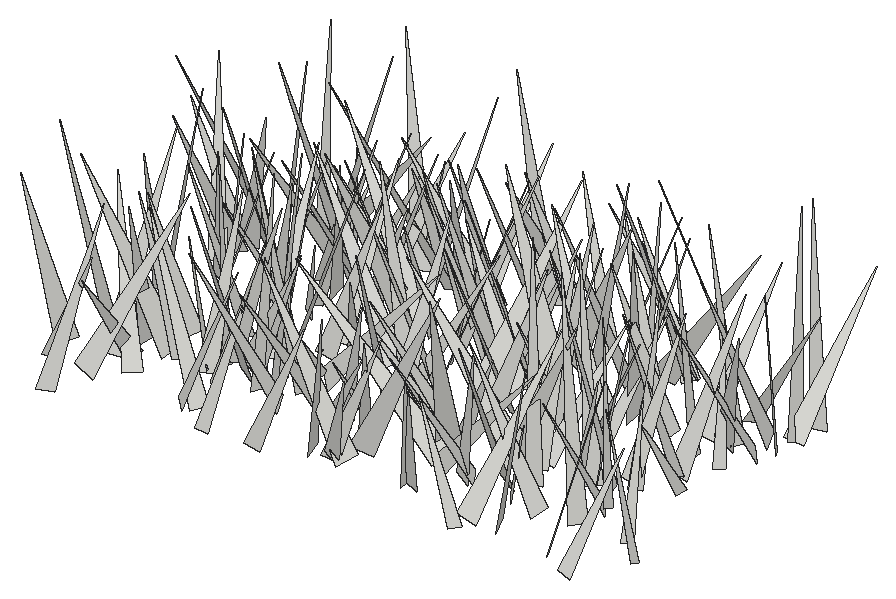
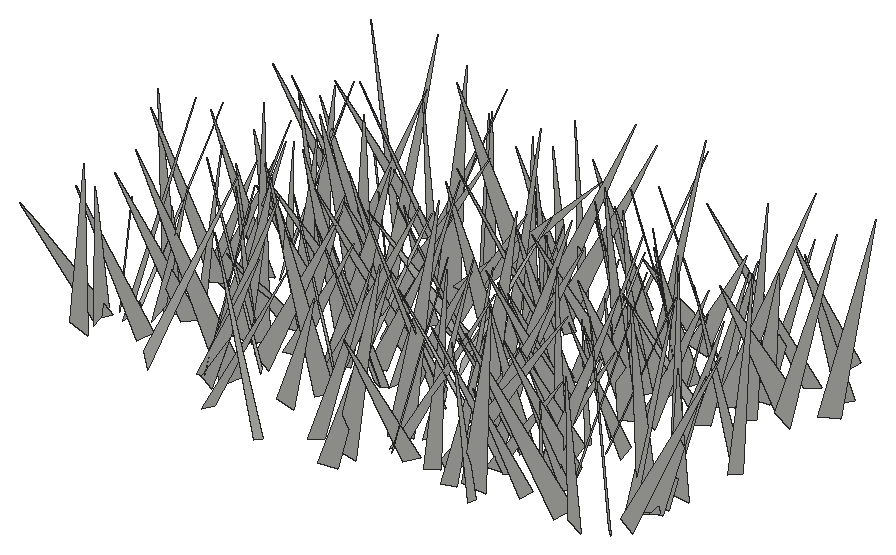
# SketchUp Ruby script. Lengths in inches.
U = 1.inch
M = Sketchup.active_model
def pt(a) = Geom::Point3d.new(a.map { |v| v * U })
def face(e, loops, mat)
  f = e.add_face(loops[0].map { |a| pt(a) })
  loops[1..].each { |l| e.add_face(l.map { |a| pt(a) }).erase! }
  f.material = f.back_material = mat if mat
  f
end
# faces: each face lists its corners as indices into pts; further lists are holes
def faces(e, pts, list, mat = nil) = list.each { |f| face(e, (f[0].is_a?(Array) ? f : [f]).map { |l| l.map { |i| pts[i] } }, mat) }
# xy, xz, yz: faces in a plane at the given z, y or x. An outline is a flat list of corners, or four numbers for a rectangle; further outlines are holes
def ring(l) = l.size == 4 ? [[l[0], l[1]], [l[2], l[1]], [l[2], l[3]], [l[0], l[3]]] : l.each_slice(2).to_a
def flat(e, list, mat, &to3) = list.each { |f| face(e, (f[0].is_a?(Array) ? f : [f]).map { |l| ring(l).map { |u, v| to3.(u, v) } }, mat) }
def xy(e, z, list, mat = nil) = flat(e, list, mat) { |x, y| [x, y, z] }
def xz(e, y, list, mat = nil) = flat(e, list, mat) { |x, z| [x, y, z] }
def yz(e, x, list, mat = nil) = flat(e, list, mat) { |y, z| [x, y, z] }
def lines(e, pts, list) = list.each { |a, b| e.add_line(pt(pts[a]), pt(pts[b])) }
# prism: a flat outline (further loops are holes) pulled along v
def prism(e, loops, v, mat = nil)
  f = face(e, loops, mat); d = Geom::Vector3d.new(v.map { |x| x * U })
  f.pushpull(f.normal.samedirection?(d) ? d.length : -d.length)
end
def box(e, o, s, mat = nil) = prism(e, [[o, [o[0] + s[0], o[1], o[2]], [o[0] + s[0], o[1] + s[1], o[2]], [o[0], o[1] + s[1], o[2]]]], [0, 0, s[2]], mat)
def at(x, y, z, deg = 0) = Geom::Transformation.translation(pt([x, y, z])) * Geom::Transformation.rotation(ORIGIN, Z_AXIS, deg.degrees)
def axes(o, x, y, z) = Geom::Transformation.new([*x, 0, *y, 0, *z, 0, *pt(o).to_a, 1])
def part(name) = M.definitions.add(name)
# library, detail: a bought-in or finely detailed component or shape, given as its bounding box
def library(name, o, s) = part(name).tap { |d| box(d.entities, o, s) }
def detail(e, o, s) = box(e.add_group.entities, o, s)
def put(e, d, t, mat = nil) = e.add_instance(d, t).tap { |i| i.material = mat if mat }
def group(e, t, mat = nil) = e.add_group.tap { |g| g.transformation = t; g.material = mat if mat }.entities
root = M.entities
c1 = part("fur_instance\#9")
p = [[0.8125,0,1.79],[0.67,-0.02,1.48],[0,-0.11,0],[0,0.11,0]]
faces(c1.entities,p,[[0,1,2,3]])
put(root,c1,axes([472.82,384.25,-21.66],[2.29321,-4.71361,1.70331],[-4.8602,-1.63403,2.02152],[1.22385,2.34308,4.83635]))
put(root,c1,axes([457.65,381.76,-21.66],[-5.19171,3.73852,1.55221],[3.028,5.26206,-2.54592],[2.68647,1.29382,5.8693]))
put(root,c1,axes([477.86,386.23,-21.66],[0.93957,-4.99379,0.05949],[-4.70596,-0.86502,1.71172],[1.67197,0.37157,4.78443]))
put(root,c1,axes([489.8,384.13,-21.66],[-1.66543,4.2087,0.7623],[4.0491,1.28782,1.73616],[-1.37806,-1.30242,4.18002]))
put(root,c1,axes([484.14,386.64,-21.66],[-0.53016,-5.209,0.61736],[-4.97847,0.69512,1.58982],[1.65216,0.4231,4.98871]))
put(root,c1,axes([455.08,385.44,-21.66],[2.87453,-4.20489,0.68169],[-4.14129,-2.56592,1.63539],[0.99777,1.46412,4.82385]))
put(root,c1,axes([499.25,383.7,-21.66],[0.30593,5.01742,0.69432],[4.86404,-0.09691,-1.44288],[1.4134,-0.75252,4.8152]))
put(root,c1,axes([476.16,386.43,-21.66],[6.10646,0.88523,1.50787],[1.27518,-6.00248,-1.64024],[-1.19633,-1.87958,5.94829]))
put(root,c1,axes([483.65,386.91,-21.66],[5.31663,-1.02418,0.76649],[-0.77202,-5.18142,-1.56841],[-1.02002,-1.41668,5.18224]))
put(root,c1,axes([491.88,386.17,-21.66],[6.71325,2.37054,1.67819],[2.73448,-6.58312,-1.63968],[-0.97898,-2.13225,6.9281]))
put(root,c1,axes([459.37,388.86,-21.66],[4.70734,-3.12135,0.14145],[-2.64852,-4.12178,-2.81392],[-1.65776,-2.27815,4.89732]))
put(root,c1,axes([478.77,386.71,-21.66],[-7.28796,2.50197,0.93453],[2.66483,6.99355,2.0583],[0.17855,-2.25345,7.42547]))
put(root,c1,axes([465.61,385.81,-21.66],[4.35224,4.23695,0.82253],[4.28263,-4.09432,-1.57033],[0.53605,-1.68972,5.86752]))
put(root,c1,axes([454.67,387.77,-21.66],[4.91943,-4.73173,2.30235],[-4.40019,-5.42749,-1.75256],[-2.8859,0.2095,6.59686]))
put(root,c1,axes([476.04,389.46,-21.66],[2.18391,-6.70079,0.42323],[-6.08063,-2.16263,-2.86325],[-2.84706,-0.52116,6.43986]))
put(root,c1,axes([477.76,386.2,-21.66],[2.95683,-4.48742,1.40063],[-4.613,-2.45121,1.88504],[0.90496,2.16707,5.03253]))
put(root,c1,axes([486.67,390.1,-21.66],[-5.64756,-4.03637,0.24701],[-3.60758,5.22048,2.82493],[1.82721,-2.16853,6.3409]))
put(root,c1,axes([470.7,389.86,-21.66],[-6.78403,-3.28205,0.63683],[-2.89291,6.48484,2.60352],[1.67585,-2.09175,7.07224]))
put(root,c1,axes([488.67,390.94,-21.66],[-2.64275,-7.72517,0.10148],[-7.35563,2.5487,2.46402],[2.36287,-0.70608,7.78402]))
put(root,c1,axes([468.89,383.9,-21.66],[-4.90566,2.32822,0.51514],[1.6552,4.17303,-3.098],[1.71648,2.62995,4.45965]))
put(root,c1,axes([458,385.3,-21.66],[0.84349,7.5995,0.98427],[7.14395,-0.42161,-2.86687],[2.77222,-1.22577,7.08837]))
put(root,c1,axes([477.97,389.6875,-21.66],[0.06322,-6.05576,0.15688],[-5.74231,-0.00994,1.93043],[1.92942,0.16885,5.74018]))
put(root,c1,axes([496.73,385.18,-21.66],[5.00084,3.55671,0.83126],[3.26277,-4.98345,1.69387],[-1.6418,0.92989,5.89825]))
put(root,c1,axes([466.95,386.1,-21.66],[-1.95645,6.57203,0.15793],[5.85701,1.66776,3.15567],[-2.98529,-1.03499,6.08778]))
put(root,c1,axes([478.7,388.26,-21.66],[4.47531,-6.51665,1.20055],[-6.35255,-3.80729,3.0143],[1.88498,2.64087,7.30815]))
put(root,c1,axes([492.91,389.04,-21.66],[-6.35837,1.48,1.02188],[1.69793,6.17763,1.61781],[0.593,-1.81932,6.3247]))
put(root,c1,axes([489.7,385.46,-21.66],[0.36828,7.38641,0.21711],[7.15433,-0.30198,-1.86176],[1.84979,-0.30261,7.15741]))
put(root,c1,axes([486.15,389.51,-21.66],[-1.36067,-5.7583,1.83351],[-5.61411,1.9,1.80082],[2.23642,1.26617,5.63617]))
put(root,c1,axes([466.64,391.48,-21.66],[-3.41876,-7.6362,0.72671],[-7.48826,3.49493,1.49637],[1.66304,0.03883,8.23167]))
put(root,c1,axes([490.25,389.39,-21.66],[3.23905,1.92957,1.10614],[2.22288,-2.8741,-1.49551],[-0.07469,-1.85863,3.46094]))
put(root,c1,axes([474.83,389.55,-21.66],[1.43751,-4.12245,0.23292],[-3.7226,-1.18725,1.96162],[1.78636,0.84328,3.90039]))
put(root,c1,axes([460.84,390.97,-21.66],[-7.92224,1.63819,2.17065],[2.33717,7.51957,2.85498],[1.39032,-3.306,7.56932]))
put(root,c1,axes([458.68,391.3125,-21.66],[6.56004,-2.8558,0.90961],[-2.50702,-6.42798,-2.10074],[-1.6425,-1.59457,6.83935]))
put(root,c1,axes([483.9,390.02,-21.66],[5.26826,5.58359,0.80335],[4.69893,-3.73546,-4.8521],[3.1212,-3.80083,5.9488]))
put(root,c1,axes([465.9,388.77,-21.66],[4.67492,4.49227,1.13099],[4.6277,-4.45606,-1.42912],[0.20972,-1.8104,6.324]))
put(root,c1,axes([483.08,392.04,-21.66],[6.31463,-5.10403,0.36931],[-4.97216,-6.25818,-1.47472],[-1.21044,-0.91981,7.98441]))
put(root,c1,axes([460.55,387.125,-21.66],[-2.20757,6.36235,0.08993],[6.1827,2.12231,1.62203],[-1.50393,-0.61421,6.5362]))
put(root,c1,axes([501.91,387.74,-21.66],[-5.07583,-0.99149,0.0646],[-0.93064,4.62637,-2.11704],[-0.34804,2.08923,4.7186]))
put(root,c1,axes([495.84,392.17,-21.66],[-4.51609,-3.87484,0.43498],[-3.47065,4.29803,2.25393],[1.77713,-1.453,5.5072]))
put(root,c1,axes([477.19,391.42,-21.66],[-3.37323,-1.69913,0.74168],[-1.13548,3.11072,1.96213],[1.46554,-1.50074,3.22735]))
put(root,c1,axes([456.77,389.98,-21.66],[-2.69995,-7.06667,2.40673],[-7.39529,2.18224,-1.88876],[-1.01973,2.88442,7.32531]))
put(root,c1,axes([474.93,391.46,-21.66],[0.27487,-5.90315,0.86813],[-5.62576,0.03312,2.00651],[1.98787,0.91,5.55848]))
put(root,c1,axes([483.4,390.86,-21.66],[-5.86481,5.71927,0.12396],[4.62698,4.63811,4.91939],[-3.36399,-3.59156,6.55024]))
put(root,c1,axes([461.88,390.52,-21.66],[-1.46223,5.38545,2.28823],[5.73287,0.84616,1.67196],[-1.17188,-2.58033,5.32407]))
put(root,c1,axes([493.32,392.2,-21.66],[-0.9776,-5.25666,1.94415],[-5.10339,1.65068,1.89699],[2.31681,1.41798,4.99896]))
put(root,c1,axes([499.82,389.61,-21.66],[-4.30895,1.90574,0.59057],[1.67064,4.21479,-1.41144],[1.09067,1.07302,4.49519]))
put(root,c1,axes([467.54,391.4,-21.66],[3.43659,4.37627,1.35344],[4.55407,-3.08156,-1.59944],[0.49399,-2.03617,5.32951]))
put(root,c1,axes([464.3125,390.48,-21.66],[-4.28089,-1.18354,0.47624],[-1.27514,3.91753,-1.72642],[-0.03977,1.79046,4.09221]))
put(root,c1,axes([476.07,394.37,-21.66],[-2.59583,-7.17613,0.91864],[-6.91744,2.74775,1.9178],[2.11891,0.17907,7.38629]))
put(root,c1,axes([495.76,389.51,-21.66],[-8.22184,1.12863,0.67504],[0.91948,7.98903,-2.15825],[0.94024,2.05661,8.01339]))
put(root,c1,axes([465.83,392.55,-21.66],[0.54416,-5.67013,1.84078],[-5.27926,0.40028,2.79359],[2.76917,1.87733,4.9641]))
put(root,c1,axes([470.54,394.35,-21.66],[3.27584,-2.78093,0.2499],[-2.38988,-2.99185,-1.96583],[-1.44378,-1.35736,3.82103]))
put(root,c1,axes([464.33,390.125,-21.66],[-4.85985,3.92503,1.53679],[3.59209,5.08366,-1.6245],[2.20555,0.36911,6.032]))
put(root,c1,axes([468.42,390.41,-21.66],[-7.01527,0.64484,2.20419],[0.06996,7.14138,-1.86657],[2.29551,1.75305,6.79307]))
put(root,c1,axes([457.87,388.16,-21.66],[-6.65412,4.03174,0.74119],[3.28122,6.08544,-3.64454],[2.45722,2.79179,6.87384]))
put(root,c1,axes([464.7,392.25,-21.66],[5.22316,-4.20753,1.34718],[-4.41725,-5.01042,1.47756],[-0.07792,1.998,6.54228]))
put(root,c1,axes([460.52,393.67,-21.66],[-5.0365,1.95588,2.0654],[2.56555,4.93734,1.5806],[1.22852,-2.29236,5.16658]))
put(root,c1,axes([481.3125,394.34,-21.66],[0.83306,-5.07313,1.39633],[-4.3947,-1.44829,-2.63999],[-2.89363,0.73905,4.41148]))
put(root,c1,axes([469.78,390.22,-21.66],[4.59054,6.55576,1.84003],[6.00661,-4.94402,2.62946],[-3.20693,0.124,7.5589]))
put(root,c1,axes([486.77,394,-21.66],[2.93254,-6.52755,1.0505],[-6.19008,-2.30697,2.94501],[2.32281,2.09313,6.52193]))
put(root,c1,axes([464.77,391.67,-21.66],[-6.75602,-0.97126,1.58692],[-1.43223,6.52998,-2.10085],[1.1876,2.34979,6.49412]))
put(root,c1,axes([464.48,391.13,-21.66],[5.18637,5.57386,2.23152],[5.04396,-5.64447,2.37581],[-3.2567,0.13438,7.23339]))
put(root,c1,axes([470.87,391.87,-21.66],[-7.866,-1.33504,0.19154],[-1.32695,7.45779,-2.51268],[-0.24134,2.50839,7.5725]))
put(root,c1,axes([486.14,394.83,-21.66],[-7.10232,2.48969,0.17848],[2.39972,6.66255,2.55443],[-0.68683,-2.46683,7.07929]))
put(root,c1,axes([482.45,394.32,-21.66],[1.69765,-3.69471,0.41656],[-3.54176,-1.46758,1.41724],[1.13153,0.9496,3.81108]))
put(root,c1,axes([470.97,394.23,-21.66],[5.03462,6.0848,0.40692],[5.07887,-3.8915,-4.64748],[3.37572,-3.22012,6.38538]))
put(root,c1,axes([478.5625,395.4,-21.66],[-4.09373,-0.36711,0.23804],[-0.24891,3.79616,1.57392],[0.35983,-1.55061,3.79686]))
put(root,c1,axes([490.3,391.76,-21.66],[1.13757,8.04859,1.54719],[7.76789,-1.55698,2.3882],[-2.61411,-1.12413,7.76984]))
put(root,c1,axes([487.18,392.28,-21.66],[-2.89965,3.32427,1.06428],[2.78447,3.03733,-1.90073],[2.1048,0.5615,3.98069]))
put(root,c1,axes([496,392.39,-21.66],[-6.18556,-0.57175,1.0735],[-0.94708,5.75521,-2.39186],[0.76312,2.5082,5.73298]))
put(root,c1,axes([468.7,392.64,-21.66],[-4.6642,0.46344,0.8289],[0.1067,4.38406,-1.85075],[0.94364,1.79496,4.30631]))
put(root,c1,axes([464.67,396.26,-21.66],[0.15208,-7.64456,1.76209],[-7.47072,0.39677,2.36609],[2.3943,1.72356,7.27077]))
put(root,c1,axes([494.63,394.7,-21.66],[-7.44301,-3.63877,0.95843],[-3.76282,7.20814,-1.85509],[0.01898,2.08796,8.0745]))
put(root,c1,axes([469.61,393.62,-21.66],[-7.1733,-2.93015,0.73361],[-2.97558,6.52972,-3.01478],[-0.51951,3.05896,7.13815]))
put(root,c1,axes([498.42,396.97,-21.66],[2.63611,-2.6678,0.56163],[-2.26437,-2.5776,-1.61563],[-1.51829,-0.78771,3.38467]))
put(root,c1,axes([489.14,393.42,-21.66],[-5.55671,4.70477,2.20019],[4.40361,5.97611,-1.65743],[2.7539,-0.06297,7.08977]))
put(root,c1,axes([470.57,397.75,-21.66],[5.43533,-0.93824,0.08866],[-0.80913,-4.91198,-2.3767],[-0.48317,-2.32876,4.97739]))
put(root,c1,axes([454.73,397.4375,-21.66],[6.40589,-1.32849,1.4611],[-0.83624,-6.31798,-2.07823],[-1.78897,-1.80373,6.20333]))
put(root,c1,axes([463.44,395.63,-21.66],[-0.2537,5.53184,2.90433],[5.7111,-0.97344,2.35297],[-2.53371,-2.74807,5.0129]))
put(root,c1,axes([469.34,391.5625,-21.66],[6.78257,3.66457,1.14232],[2.83952,-6.35069,3.51329],[-2.58286,2.6414,6.86216]))
put(root,c1,axes([462.27,392.2,-21.66],[5.32818,4.49942,0.50618],[3.89144,-4.95023,3.04014],[-2.31467,2.03493,6.2763]))
put(root,c1,axes([493.37,394.1,-21.66],[-7.58228,1.17889,0.51367],[1.00041,7.33787,-2.07353],[0.80796,1.97752,7.38791]))
put(root,c1,axes([476.41,394.98,-21.66],[-2.09917,6.50868,2.06271],[6.47308,2.58358,-1.56477],[2.17184,-1.40938,6.65739]))
put(root,c1,axes([493.51,394.16,-21.66],[3.73526,4.02595,0.93613],[3.5763,-3.78049,1.98866],[-2.07237,0.73241,5.11915]))
put(root,c1,axes([489.04,394.6,-21.66],[-0.72981,5.66267,0.18679],[5.27184,0.7477,-2.06932],[2.0757,0.09199,5.32132]))
put(root,c1,axes([468.97,396.73,-21.66],[2.35297,-5.60644,2.50548],[-6.03434,-1.6135,2.05656],[1.13856,3.03489,5.72182]))
put(root,c1,axes([494.92,396.01,-21.66],[0.03903,6.40601,1.64221],[6.43648,0.34027,-1.48032],[1.51842,-1.60705,6.23275]))
put(root,c1,axes([491.09,395.7,-21.66],[4.64309,0.99306,0.50279],[0.80416,-4.48393,1.43003],[-0.7696,1.30595,4.52764]))
put(root,c1,axes([456.37,395.5,-21.66],[6.51752,3.06728,2.32468],[2.5593,-6.86862,1.88745],[-2.87443,0.8392,6.95153]))
put(root,c1,axes([466.09,394.17,-21.66],[-5.16112,5.15909,0.10388],[4.87926,4.92701,-2.27629],[1.67923,1.54029,6.93338]))
put(root,c1,axes([463.09,400.33,-21.66],[-4.74866,-3.13825,0.27488],[-2.86364,4.50737,1.98925],[1.31291,-1.51952,5.33303]))
put(root,c1,axes([483.28,398.32,-21.66],[-3.66042,-4.84933,0.70173],[-4.78346,3.34689,-1.82316],[-1.06154,1.63996,5.79575]))
put(root,c1,axes([482.21,397.54,-21.66],[1.25839,-5.65908,2.69216],[-6.0262,-0.33916,2.10388],[1.71982,2.95233,5.40207]))
put(root,c1,axes([477.375,397.82,-21.66],[-7.14593,-4.06809,0.00282],[-3.91681,6.87864,-2.22635],[-1.09909,1.93614,7.91562]))
put(root,c1,axes([476.01,397.3,-21.66],[3.46284,5.45761,0.55951],[5.19477,-3.049,-2.40992],[1.76435,-1.73432,5.99742]))
put(root,c1,axes([457.36,400.3,-21.66],[-1.15928,-6.64992,1.1524],[-6.36185,1.46707,2.06591],[2.25307,0.72087,6.42631]))
put(root,c1,axes([486.22,399.79,-21.66],[-4.22859,-0.79072,0.99748],[-0.41595,4.12901,1.5098],[1.20299,-1.35177,4.02824]))
put(root,c1,axes([495.81,395.41,-21.66],[-6.32088,1.55628,0.92222],[1.03646,5.86264,-2.78949],[1.48264,2.53644,5.88169]))
put(root,c1,axes([496.86,398.52,-21.66],[-1.92463,-5.23066,1.71698],[-5.26178,1.21283,-2.20335],[-1.6191,2.27625,5.1195]))
put(root,c1,axes([474.71,398.29,-21.66],[-1.73257,6.85044,2.42635],[7.20837,1.30251,1.46979],[-0.92468,-2.68187,6.91158]))
put(root,c1,axes([464.72,400.32,-21.66],[-1.05562,-3.90874,0.84941],[-3.49411,1.32871,1.77194],[1.94702,0.26528,3.64044]))
put(root,c1,axes([473.16,398.65,-21.66],[-5.71693,5.39586,0.3581],[5.20349,5.34707,2.50186],[-1.47216,-2.05434,7.45247]))
put(root,c1,axes([478.94,394.9,-21.66],[6.66219,5.05954,0.23915],[4.47229,-6.06129,3.64695],[-2.37798,2.77537,7.52884]))
put(root,c1,axes([486.45,398.26,-21.66],[6.53232,-2.04401,3.08815],[-2.89411,-6.72439,1.67109],[-2.31057,2.64395,6.63752]))
put(root,c1,axes([464.46,398.28,-21.66],[3.7445,3.22853,1.26331],[2.91821,-3.9391,1.41711],[-1.87174,0.31742,4.73672]))
put(root,c1,axes([468.5625,397.27,-21.66],[5.48783,2.36239,1.1528],[1.72376,-5.24883,2.55038],[-1.98455,1.97355,5.40302]))
put(root,c1,axes([496.82,398.58,-21.66],[0.16958,6.97336,1.46095],[6.91324,0.19239,-1.72074],[1.72314,-1.45812,6.75984]))
put(root,c1,axes([479.39,401.86,-21.66],[-7.48109,-1.28394,1.71532],[-0.94889,7.57103,1.5286],[1.92105,-1.26035,7.43496]))
put(root,c1,axes([499.0625,403.91,-21.66],[-5.37416,-4.85351,0.14678],[-4.51514,5.07548,2.5125],[1.7865,-1.77274,6.79157]))
put(root,c1,axes([482.9375,401.17,-21.66],[-5.86461,-3.9483,0.52207],[-3.9663,5.70596,-1.40208],[-0.36068,1.452,6.92942]))
put(root,c1,axes([496.57,403.71,-21.66],[-0.05965,-7.49908,0.31223],[-6.76708,0.1888,3.24163],[3.24657,0.25574,6.76251]))
put(root,c1,axes([493.22,402.39,-21.66],[-6.6748,0.96554,1.83268],[1.43583,6.61336,1.7452],[1.49311,-2.0433,6.51456]))
put(root,c1,axes([489.83,402.99,-21.66],[7.80174,-0.94154,1.76979],[-0.49694,-7.7978,-1.95786],[-1.94209,-1.78708,7.61055]))
put(root,c1,axes([469.38,404.48,-21.66],[6.1806,-4.85252,1.92283],[-3.89661,-6.27237,-3.30423],[-3.47285,-1.59827,7.12944]))
put(root,c1,axes([468.61,398.66,-21.66],[-3.2571,5.60614,0.8435],[5.30317,3.35677,-1.83235],[2.00417,0.22864,6.21933]))
put(root,c1,axes([462.03,399.73,-21.66],[5.46763,0.70402,1.09334],[0.38726,-5.3924,1.5356],[-1.2414,1.41859,5.29457]))
put(root,c1,axes([455.94,403.9,-21.66],[2.22572,-6.24997,0.53761],[-6.03536,-2.28904,-1.62473],[-1.71046,-0.05581,6.43243]))
put(root,c1,axes([481.73,401.01,-21.66],[-4.33384,4.15795,0.46311],[4.09626,4.08164,1.68703],[-0.85069,-1.52868,5.76409]))
put(root,c1,axes([472.49,403.5,-21.66],[5.01646,-0.03484,2.02413],[0.79085,-4.94522,-2.0451],[-1.86357,-2.19241,4.58078]))
put(root,c1,axes([467.9,398.24,-21.66],[7.02675,2.35333,1.41841],[1.60681,-6.67867,3.12071],[-2.22895,2.60433,6.72121]))
put(root,c1,axes([488.88,400.375,-21.66],[-3.57557,6.64036,0.56629],[6.42877,3.26724,2.27945],[-1.75672,-1.55901,7.1891]))
put(root,c1,axes([464.4,403.55,-21.66],[6.47505,-0.26988,1.20187],[0.07267,-6.33614,-1.81428],[-1.22965,-1.79557,6.22153]))
put(root,c1,axes([479.98,398.87,-21.66],[0.04279,8.23701,0.26485],[7.98617,0.02394,-2.03491],[2.0346,-0.26721,7.98181]))
put(root,c1,axes([484.01,402.25,-21.66],[-5.61004,5.72169,2.32507],[6.16954,5.3361,1.75473],[0.28367,-2.89906,7.81865]))
put(root,c1,axes([496.12,401.23,-21.66],[-7.03444,-1.19576,1.59787],[-1.52444,6.99776,-1.47438],[1.28808,1.75153,6.98136]))
put(root,c1,axes([490.02,399.64,-21.66],[-3.33289,3.23483,0.32122],[2.5841,2.91556,-2.549],[1.97223,1.64647,3.88264]))
put(root,c1,axes([478.18,402.39,-21.66],[-1.48445,-5.73193,2.26963],[-5.6541,0.33538,-2.85107],[-2.45713,2.69116,5.18942]))
put(root,c1,axes([479.74,402.65,-21.66],[2.31497,4.33574,1.17317],[4.28428,-1.73503,-2.04175],[1.34907,-1.93005,4.47091]))
put(root,c1,axes([498.38,400.98,-21.66],[-4.64664,1.60589,0.29185],[1.45378,4.47236,-1.46283],[0.74202,1.29401,4.69365]))
put(root,c1,axes([460.67,407.74,-21.66],[-6.33754,-5.19611,0.8236],[-4.02771,5.62162,4.47406],[3.3846,-3.03975,6.86635]))
put(root,c1,axes([498.58,406,-21.66],[-6.83559,-3.49227,1.59422],[-2.83471,6.78714,2.71329],[2.5888,-1.7893,7.18049]))
put(root,c1,axes([456.85,405.6875,-21.66],[-3.15588,-6.30761,0.73503],[-6.08642,3.23856,1.65924],[1.81157,-0.10755,6.85511]))
put(root,c1,axes([467.08,403.61,-21.66],[3.19208,-3.97574,0.46961],[-3.91795,-2.97897,1.41133],[0.82265,1.2392,4.89939]))
put(root,c1,axes([483.3,403.86,-21.66],[-3.35024,-7.10363,1.41562],[-6.97339,2.74138,-2.74705],[-1.95891,2.39017,7.35795]))
put(root,c1,axes([475.38,402.32,-21.66],[3.97232,6.71602,1.21655],[6.692,-3.55551,-2.22255],[1.34242,-2.14887,7.47961]))
put(root,c1,axes([487.2,402.96,-21.66],[-4.10469,4.34568,0.4298],[4.19686,3.76273,2.03626],[-1.20665,-1.6956,5.62024]))
put(root,c1,axes([480.36,402.66,-21.66],[3.62784,4.7769,0.79864],[4.78599,-3.38301,-1.50576],[0.74217,-1.53438,5.80626]))
put(root,c1,axes([482.87,403.77,-21.66],[5.29628,3.42643,1.15131],[3.61426,-4.98862,-1.7797],[0.0553,-2.11891,6.05175]))
put(root,c1,axes([455.875,405.06,-21.66],[2.61473,-6.42495,0.46001],[-6.33227,-2.47287,1.45453],[1.18065,0.96609,6.78241]))
put(root,c1,axes([476.03,400.94,-21.66],[3.78632,3.0497,0.88341],[2.42458,-3.66486,2.25998],[-2.05,1.29824,4.30457]))
put(root,c1,axes([487.13,401.2,-21.66],[-7.34355,0.30763,3.29021],[-0.75169,7.65215,-2.39318],[3.21793,2.48952,6.94946]))
put(root,c1,axes([464.78,405.56,-21.66],[-1.76635,-5.02439,0.02248],[-4.81779,1.68692,-1.51928],[-1.42615,0.52421,5.10454]))
put(root,c1,axes([491.2,403.52,-21.66],[-2.35431,6.5098,1.98677],[6.74258,1.94391,1.62058],[-0.92858,-2.38982,6.73008]))
put(root,c1,axes([455.63,404.8,-21.66],[-4.26864,3.3889,1.68719],[3.78174,3.93314,1.66776],[0.17248,-2.36607,5.18889]))
put(root,c1,axes([455.63,402.17,-21.66],[-1.06159,6.87885,0.56166],[6.76624,0.92524,1.45707],[-1.36093,-0.76575,6.80607]))
put(root,c1,axes([474.82,407.17,-21.66],[5.51708,-5.76072,0.82028],[-5.55442,-5.55067,-1.6234],[-1.73412,-0.54876,7.80952]))
put(root,c1,axes([464.41,401.61,-21.66],[5.42,0.95377,1.93695],[-0.10115,-5.11614,2.80228],[-2.15667,2.63692,4.73638]))
put(root,c1,axes([473.36,406.1,-21.66],[-6.08575,-1.31512,1.93305],[-0.80976,6.24223,1.69745],[2.19329,-1.34444,5.99037]))
put(root,c1,axes([488.09,405.03,-21.66],[-2.1287,-6.56011,1.58213],[-6.38568,1.42177,-2.69649],[-2.18201,2.23898,6.34786]))
put(root,c1,axes([482.17,405.85,-21.66],[1.4912,-7.63112,1.5604],[-7.07021,-0.65953,3.53123],[3.26816,2.05513,6.92734]))
put(root,c1,axes([490.82,402.5,-21.66],[3.07038,6.62387,1.59445],[6.28566,-3.42873,2.13997],[-2.62838,-0.46188,6.98022]))
put(root,c1,axes([470.73,404.26,-21.66],[-4.85114,5.94494,0.47809],[5.69058,4.42924,2.66526],[-1.78556,-2.03568,7.19529]))
put(root,c1,axes([464.12,405.69,-21.66],[1.30343,6.50873,4.51627],[7.0846,-3.00591,2.28737],[-3.54523,-3.61388,6.23141]))
put(root,c1,axes([487.41,405.91,-21.66],[6.19787,3.91116,1.13836],[4.069,-5.84754,-2.06304],[0.19042,-2.34857,7.0324]))
put(root,c1,axes([455.95,407.21,-21.66],[-2.71774,-6.73125,0.47193],[-6.54696,2.5072,-1.9416],[-1.63394,1.15011,6.99472]))
put(root,c1,axes([468.02,402.91,-21.66],[5.42222,1.22065,1.50489],[0.3801,-5.05507,2.73075],[-1.90005,2.47215,4.84081]))
put(root,c1,axes([495.1,403.65,-21.66],[-1.51128,6.4389,0.97646],[6.11666,1.74753,-2.05657],[2.23592,-0.42848,6.28601]))
put(root,c1,axes([500.01,404.84,-21.66],[-4.46035,-2.40279,1.6408],[-2.85913,4.17643,-1.65628],[0.53948,2.26814,4.788]))
put(root,c1,axes([497.35,404.19,-21.66],[-7.36083,-0.13148,0.37404],[-0.23398,7.05478,-2.12469],[0.32007,2.13349,7.04874]))
put(root,c1,axes([490.09,408.33,-21.66],[-5.41835,-3.58553,1.38238],[-3.2455,5.54933,1.6725],[2.0576,-0.68883,6.27832]))
put(root,c1,axes([467.46,406.71,-21.66],[-3.75948,2.94392,0.27379],[2.73653,3.29698,2.12525],[-1.1194,-1.82718,4.27594]))
put(root,c1,axes([461.97,405.95,-21.66],[0.15011,3.96157,1.30257],[3.86973,0.35348,-1.52101],[1.55431,-1.26265,3.66102]))
put(root,c1,axes([474.12,408.83,-21.66],[-5.52668,-3.91053,1.22579],[-3.5737,5.60606,1.77193],[2.00587,-0.78663,6.53427]))
put(root,c1,axes([470.54,409.2,-21.66],[0.16634,-6.6201,0.01552],[-6.42128,-0.15757,1.61124],[1.61035,0.05552,6.42319]))
put(root,c1,axes([474.13,408.33,-21.66],[-7.00038,0.48524,0.02911],[0.47648,6.76613,1.79834],[-0.09628,-1.796,6.78283]))
put(root,c1,axes([471.55,403.22,-21.66],[5.15692,6.28398,0.1894],[5.87834,-4.90651,2.73667],[-2.22922,1.59869,7.6546]))
put(root,c1,axes([487.97,408.08,-21.66],[4.31656,-7.06636,0.27005],[-6.24466,-3.6606,4.0303],[3.31821,2.3034,7.23345]))
put(root,c1,axes([463.9,406.11,-21.66],[1.76698,3.75792,1.11012],[3.4505,-2.06932,1.51278],[-1.85698,-0.26926,3.86726]))
put(root,c1,axes([496.09,407.17,-21.66],[4.90095,-2.69617,0.00541],[-2.57457,-4.67657,1.67032],[0.80058,1.46597,5.33842]))
put(root,c1,axes([456.32,408.48,-21.66],[5.45903,4.38742,2.52703],[5.0114,-5.21201,-1.77686],[-0.72192,-3.00365,6.77446]))
put(root,c1,axes([469.76,408.72,-21.66],[-3.41379,-7.32141,0.63154],[-6.65452,2.7845,-3.69049],[-3.11756,2.07349,7.18591]))
put(root,c1,axes([489.42,409.25,-21.66],[-2.75065,-6.97463,1.22589],[-6.99898,2.47729,-1.60986],[-1.07823,1.71227,7.32256]))
put(root,c1,axes([462.47,404.32,-21.66],[-6.96158,0.42843,3.50828],[-1.43896,6.73486,-3.67782],[3.22816,3.92599,5.92628]))
put(root,c1,axes([468.37,410.2,-21.66],[3.73723,-3.51523,0.8829],[-3.22394,-3.80362,-1.49732],[-1.65607,-0.52811,4.90732]))
put(root,c1,axes([466.13,406.64,-21.66],[1.18506,6.07091,0.5983],[5.8889,-0.9794,-1.72625],[1.5921,-0.89616,5.93973]))
put(root,c1,axes([494.11,409.53,-21.66],[-5.74525,-5.95088,0.61636],[-5.93253,5.55629,-1.65334],[-0.77329,1.58601,8.10478]))
put(root,c1,axes([460.12,408.54,-21.66],[4.62991,-4.98565,0.093],[-4.3743,-3.99984,3.34189],[2.39393,2.33366,5.92659]))
put(root,c1,axes([463.6,408.1,-21.66],[3.57113,-2.0967,0.79041],[-2.23153,-3.1932,1.61171],[0.20288,1.78359,3.81464]))
put(root,c1,axes([489.68,408.88,-21.66],[-3.57331,4.48467,0.98446],[4.4978,3.16833,1.89248],[-0.92266,-1.92337,5.41289]))
put(root,c1,axes([478.97,410.75,-21.66],[5.01755,-2.86523,2.69296],[-2.1597,-5.65647,-1.99435],[-3.28592,-0.6574,5.42291]))
put(root,c1,axes([476.15,413.07,-21.66],[4.64507,-4.79979,0.2726],[-4.36308,-4.36804,-2.56373],[-2.01887,-1.6035,6.16782]))
put(root,c1,axes([465.91,410.91,-21.66],[5.21952,0.68023,0.61562],[0.83808,-4.98198,-1.60081],[-0.37326,-1.674,5.01433]))
put(root,c1,axes([499.94,406.875,-21.66],[-7.67594,0.43258,1.18162],[-0.05572,7.18028,-2.99063],[1.25708,2.9597,7.0826]))
put(root,c1,axes([483.38,408.45,-21.66],[-1.50811,5.89701,0.63499],[5.61901,1.21081,2.10069],[-1.89858,-1.1007,5.71281]))
put(root,c1,axes([499.87,406.84,-21.66],[-2.9172,5.75801,0.16061],[5.28877,2.74872,-2.48273],[2.2824,0.99014,5.95825]))
put(root,c1,axes([487.06,411.87,-21.66],[-5.99784,0.36822,0.31916],[0.44096,5.77868,1.61988],[0.20737,-1.63795,5.78668]))
put(root,c1,axes([500.14,408.98,-21.66],[0.70044,7.59304,1.85976],[7.56257,-1.13109,1.76971],[-1.98005,-1.63401,7.41708]))
put(root,c1,axes([466.85,409.48,-21.66],[-1.50956,7.97784,1.83345],[8.07703,1.14872,1.65178],[-1.3301,-2.07864,7.94961]))
put(root,c1,axes([458.59,409.36,-21.66],[1.63726,6.8228,1.57078],[6.72877,-1.9791,1.58281],[-1.9343,-1.10957,6.83563]))
put(root,c1,axes([481.88,413.16,-21.66],[6.81977,1.54998,0.06465],[1.44583,-6.24479,-2.79788],[0.56233,-2.74155,6.40965]))
put(root,c1,axes([472.35,409.08,-21.66],[-2.22642,5.28944,0.76409],[4.89566,2.35054,-2.00661],[2.14349,0.12554,5.37668]))
put(root,c1,axes([476.19,411.21,-21.66],[-0.9931,7.68396,2.84346],[8.04191,0.36629,1.81887],[-1.56723,-2.98953,7.53135]))
